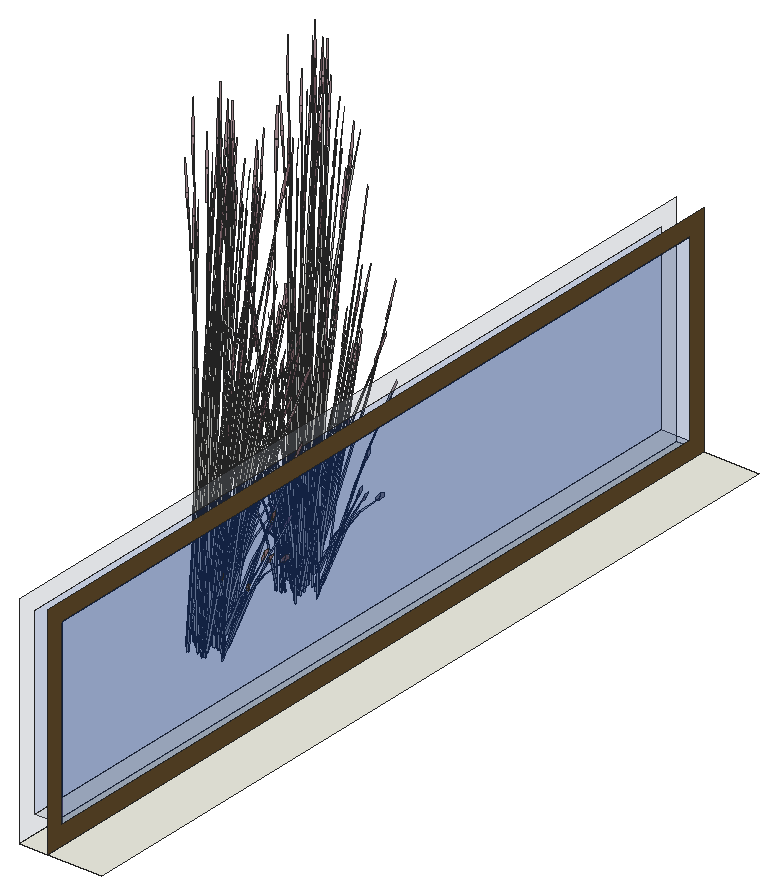
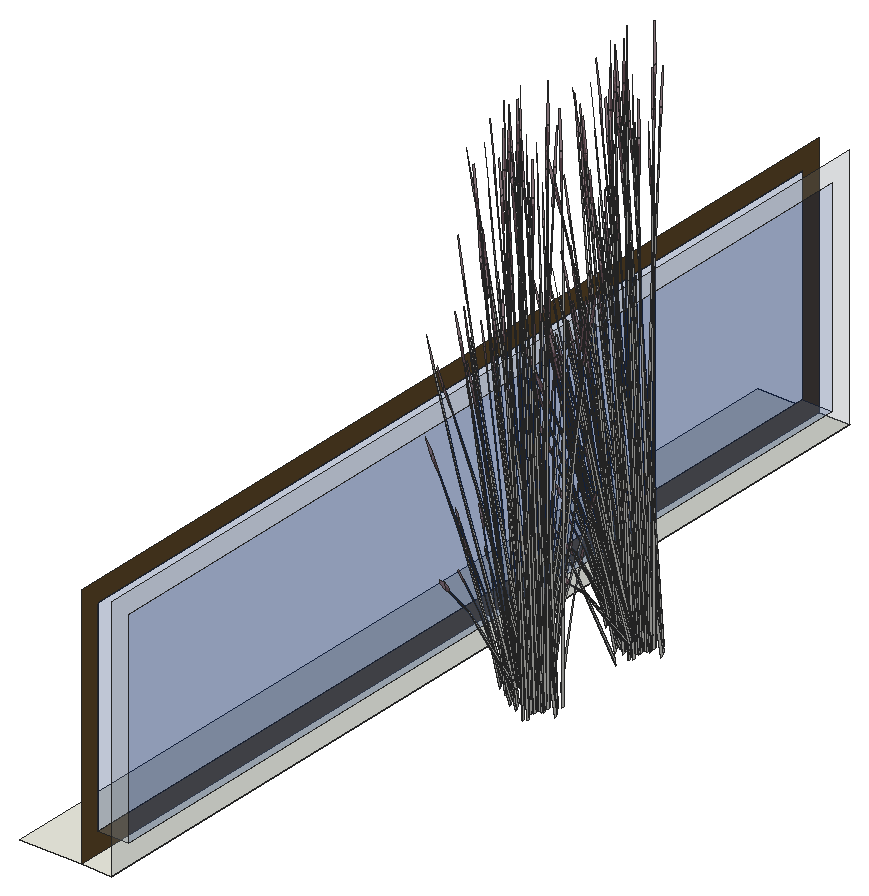
# SketchUp Ruby script. Lengths in inches.
U = 1.inch
M = Sketchup.active_model
def pt(a) = Geom::Point3d.new(a.map { |v| v * U })
def face(e, loops, mat)
  f = e.add_face(loops[0].map { |a| pt(a) })
  loops[1..].each { |l| e.add_face(l.map { |a| pt(a) }).erase! }
  f.material = f.back_material = mat if mat
  f
end
# faces: each face lists its corners as indices into pts; further lists are holes
def faces(e, pts, list, mat = nil) = list.each { |f| face(e, (f[0].is_a?(Array) ? f : [f]).map { |l| l.map { |i| pts[i] } }, mat) }
# xy, xz, yz: faces in a plane at the given z, y or x. An outline is a flat list of corners, or four numbers for a rectangle; further outlines are holes
def ring(l) = l.size == 4 ? [[l[0], l[1]], [l[2], l[1]], [l[2], l[3]], [l[0], l[3]]] : l.each_slice(2).to_a
def flat(e, list, mat, &to3) = list.each { |f| face(e, (f[0].is_a?(Array) ? f : [f]).map { |l| ring(l).map { |u, v| to3.(u, v) } }, mat) }
def xy(e, z, list, mat = nil) = flat(e, list, mat) { |x, y| [x, y, z] }
def xz(e, y, list, mat = nil) = flat(e, list, mat) { |x, z| [x, y, z] }
def yz(e, x, list, mat = nil) = flat(e, list, mat) { |y, z| [x, y, z] }
def lines(e, pts, list) = list.each { |a, b| e.add_line(pt(pts[a]), pt(pts[b])) }
# prism: a flat outline (further loops are holes) pulled along v
def prism(e, loops, v, mat = nil)
  f = face(e, loops, mat); d = Geom::Vector3d.new(v.map { |x| x * U })
  f.pushpull(f.normal.samedirection?(d) ? d.length : -d.length)
end
def box(e, o, s, mat = nil) = prism(e, [[o, [o[0] + s[0], o[1], o[2]], [o[0] + s[0], o[1] + s[1], o[2]], [o[0], o[1] + s[1], o[2]]]], [0, 0, s[2]], mat)
def at(x, y, z, deg = 0) = Geom::Transformation.translation(pt([x, y, z])) * Geom::Transformation.rotation(ORIGIN, Z_AXIS, deg.degrees)
def axes(o, x, y, z) = Geom::Transformation.new([*x, 0, *y, 0, *z, 0, *pt(o).to_a, 1])
def part(name) = M.definitions.add(name)
# library, detail: a bought-in or finely detailed component or shape, given as its bounding box
def library(name, o, s) = part(name).tap { |d| box(d.entities, o, s) }
def detail(e, o, s) = box(e.add_group.entities, o, s)
def put(e, d, t, mat = nil) = e.add_instance(d, t).tap { |i| i.material = mat if mat }
def group(e, t, mat = nil) = e.add_group.tap { |g| g.transformation = t; g.material = mat if mat }.entities
root = M.entities
M.materials.add("D01_Frost_White").color = [238, 238, 227]
M.materials.add("Glass_Basic_01").color = [161, 173, 186]
M.materials["Glass_Basic_01"].alpha = 0.25
M.materials.add("Glass_Sky Reflection_01").color = [0, 46, 142]
M.materials["Glass_Sky Reflection_01"].alpha = 0.25
M.materials.add("LightPink_Translucent").color = [144, 107, 117]
M.materials["LightPink_Translucent"].alpha = 0.75
M.materials.add("Wood_Veneer_15_1K").color = [103, 79, 44]
c1 = part("blade")
p = [[2.15,0.21,22],[0,0.17,0],[0.09,0.45,0],[2.18,0.31,22],[2.29,0.31,22],[0.38,0.45,0],
  [2.48,0.24,33],[2.49,0.24,33],[2.48,0.22,33]]
faces(c1.entities,p,[[0,1,2,3],[4,5,2,3],[6,3,4,7],[8,0,3,6]])
c2 = part("seeds")
p = [[0.3,-0.1,1.38],[-0.01,-0.03,1.59],[-0.01,-0.03,0.03],[0.14,-0.07,-0.07],[0.29,-0.03,3],[0.15,0.01,3.11]]
faces(c2.entities,p,[[0,1,2,3],[1,0,4,5]],"LightPink_Translucent")
c3 = part("blade with seeds")
put(c3.entities,c1,at(0,0,0))
put(c3.entities,c2,axes([2.4,0.25,30.99],[1.5799,-0.05474,1.17369],[-0.12525,1.92788,0.29478],[-0.07173,-0.02425,1.56792]))
xy(root,156,[[427,586,430,676],[430,586,436,676]],"D01_Frost_White")
xy(root,158,[[427,588,430,674]],"Glass_Basic_01")
yz(root,427,[[[586,156,676,180],[588,158,674,178]]],"Glass_Basic_01")
yz(root,427,[[588,158,674,178]],"Glass_Sky Reflection_01")
yz(root,430,[[588,158,674,178]],"Glass_Sky Reflection_01")
yz(root,430,[[[586,156,676,180],[588,158,674,178]]],"Wood_Veneer_15_1K")
put(root,c3,axes([417.75,623.51,155.72],[-0.19883,0.425,-0.37796],[-0.41314,-0.20454,0.1819],[0,0.09797,1.2135]))
put(root,c3,axes([417.54,634.06,158.27],[0.30197,-0.1603,0.05432],[0.1478,0.29231,0.42765],[-0.02916,-0.12885,0.65209]))
put(root,c3,axes([416.5625,625.95,157.83],[0.05195,0.07595,1.47793],[0.41921,0.02984,-0.23373],[0.04216,0.1675,0.11853]))
put(root,c3,axes([418.54,623.25,155.94],[-0.32198,-0.34356,0.14904],[0.32447,-0.33323,0.29641],[-0.03556,0.07016,1.35512]))
put(root,c3,axes([418.54,636.21,156.37],[-0.32198,-0.34356,0.14904],[0.32447,-0.33323,0.29641],[-0.03556,0.07016,1.35512]))
put(root,c3,axes([417.43,623.05,155.71],[0,-0.54574,0],[0.51243,0,0],[0,0,1.51605]))
put(root,c3,axes([417.43,636.01,156.14],[0,-0.54574,0],[0.51243,0,0],[0,0,1.51605]))
put(root,c3,axes([417.43,634.09,158.27],[0.4038,0.12331,0.40553],[-0.13808,0.40538,0.33437],[-0.02427,-0.15942,0.83914]))
put(root,c3,axes([416.95,623.15,155.91],[0.46174,0.2286,0.2033],[-0.22222,0.475,0.42242],[0,-0.1095,1.35626]))
put(root,c3,axes([416.95,636.11,156.33],[0.46174,0.2286,0.2033],[-0.22222,0.475,0.42242],[0,-0.1095,1.35626]))
put(root,c3,axes([417.68,623.27,155.79],[0,0.54548,-0.04762],[-0.51243,0,0],[0,0.01714,1.5153]))
put(root,c3,axes([417.68,636.23,156.21],[0,0.54548,-0.04762],[-0.51243,0,0],[0,0.01714,1.5153]))
put(root,c3,axes([416.8,622.83,156.15],[-0.44501,0.02912,0.37796],[-0.04024,-0.48332,-0.1819],[0.07967,-0.04899,1.2135]))
put(root,c3,axes([416.8,635.79,156.57],[-0.44501,0.02912,0.37796],[-0.04024,-0.48332,-0.1819],[0.07967,-0.04899,1.2135]))
put(root,c3,axes([416.78,624.93,158.12],[0.12355,-0.36271,0.29918],[0.36044,0.10579,-0.38624],[0.03305,0.14603,0.73904]))
put(root,c3,axes([416.59,622,155.94],[-0.11838,0.46875,0.14904],[-0.43321,-0.13265,0.29641],[0.07483,-0.00228,1.35512]))
put(root,c3,axes([416.59,634.96,156.37],[-0.11838,0.46875,0.14904],[-0.43321,-0.13265,0.29641],[0.07483,-0.00228,1.35512]))
put(root,c3,axes([417.44,624.32,155.79],[0.17817,0.54185,-0.05079],[-0.50909,0.18987,0],[0.00622,0.01892,1.45452]))
put(root,c3,axes([417.44,637.28,156.21],[0.17817,0.54185,-0.05079],[-0.50909,0.18987,0],[0.00622,0.01892,1.45452]))
put(root,c3,axes([416.38,634.38,156.28],[-0.25622,-0.47263,0],[0.42866,-0.26357,-0.43598],[0.09763,-0.06003,1.38303]))
put(root,c3,axes([416.85,624.98,158.06],[0.19559,0.38351,-0.60019],[-0.40262,0.21373,0.07243],[0.04574,0.1853,0.84903]))
put(root,c3,axes([418.91,623.61,155.71],[-0.51218,-0.00377,-0.04204],[0,-0.52715,0.42192],[-0.0161,0.12,1.33776]))
put(root,c3,axes([417.91,622.03,155.94],[-0.44036,0.12519,0.14904],[-0.10874,-0.46588,0.29641],[0.03927,0.06788,1.35512]))
put(root,c3,axes([417.91,634.99,156.37],[-0.44036,0.12519,0.14904],[-0.10874,-0.46588,0.29641],[0.03927,0.06788,1.35512]))
put(root,c3,axes([417.46,633.24,156.61],[0.05257,0.27504,0.97034],[-0.29163,-0.15233,0.71294],[0.03138,-0.14083,0.21373]))
put(root,c3,axes([417.26,626.22,158.62],[0.28319,-0.27058,-0.05481],[0.25948,0.29635,-0.2485],[0.01827,0.08397,0.81966]))
put(root,c3,axes([417.18,622.7,155.85],[-0.33979,0.42804,0.38653],[-0.40368,-0.37784,0.15168],[0.08192,-0.04272,1.34202]))
put(root,c3,axes([417.18,635.66,156.27],[-0.33979,0.42804,0.38653],[-0.40368,-0.37784,0.15168],[0.08192,-0.04272,1.34202]))
put(root,c3,axes([417.77,623.38,155.72],[0.28606,0.30466,0],[-0.28606,0.30466,0],[0,0,1.42996]))
put(root,c3,axes([417.77,636.34,156.15],[0.28606,0.30466,0],[-0.28606,0.30466,0],[0,0,1.42996]))
put(root,c3,axes([417.76,623.02,156.15],[0.19883,-0.425,0.37796],[0.41314,0.20454,-0.1819],[0,0.09797,1.2135]))
put(root,c3,axes([417.76,635.98,156.57],[0.19883,-0.425,0.37796],[0.41314,0.20454,-0.1819],[0,0.09797,1.2135]))
put(root,c3,axes([417.59,624.5,155.71],[0.41314,0.21175,0],[-0.19883,0.43999,0],[0,0,1.47801]))
put(root,c3,axes([417.59,637.46,156.14],[0.41314,0.21175,0],[-0.19883,0.43999,0],[0,0,1.47801]))
put(root,c3,axes([417,625.06,157.81],[0.40284,0.11824,-0.43168],[-0.13808,0.40538,-0.33437],[0.03694,0.16321,0.82598]))
put(root,c3,axes([416.66,625.08,158.1],[0.40102,-0.2196,-0.10273],[0.19707,0.38974,-0.57019],[0.05291,0.16424,0.8664]))
put(root,c3,axes([417.63,622.92,155.86],[-0.51796,-0.09937,0.41563],[0.10541,-0.56124,0.1631],[0.07569,0.05419,1.44303]))
put(root,c3,axes([417.63,635.88,156.29],[-0.51796,-0.09937,0.41563],[0.10541,-0.56124,0.1631],[0.07569,0.05419,1.44303]))
put(root,c3,axes([418.7,633.6875,158.25],[-0.04162,0.03603,1.49853],[-0.40776,-0.12155,-0.1416],[-0.01476,-0.15722,0.26519]))
put(root,c3,axes([418.38,634.73,158.53],[-0.45039,-0.02337,-0.10273],[0.01231,-0.44247,-0.57019],[0.03129,-0.17041,0.8664]))
put(root,c3,axes([418.8,623.6875,155.56],[-0.28606,0.29428,-0.2617],[-0.28606,-0.29428,0.2617],[0,0.09479,1.17405]))
put(root,c3,axes([417.78,623.17,155.71],[0.45849,0,0],[0,0.4883,0],[0,0,1.50718]))
put(root,c3,axes([417.78,636.13,156.14],[0.45849,0,0],[0,0.4883,0],[0,0,1.50718]))
put(root,c3,axes([418.21,634.8,158.54],[-0.27728,0.24833,0.29918],[-0.26248,-0.28355,-0.38624],[0.03994,-0.14407,0.73904]))
put(root,c3,axes([417.33,622.63,156.15],[-0.24618,-0.39589,0.37796],[0.37289,-0.27878,-0.1819],[0.07967,0.04899,1.2135]))
put(root,c3,axes([417.33,635.59,156.57],[-0.24618,-0.39589,0.37796],[0.37289,-0.27878,-0.1819],[0.07967,0.04899,1.2135]))
put(root,c3,axes([416.89,622.73,156.1],[-0.04775,-0.53819,-0.2458],[0.49736,-0.03254,-0.42242],[0.08758,-0.07169,1.34921]))
put(root,c3,axes([416.89,635.6875,156.53],[-0.04775,-0.53819,-0.2458],[0.49736,-0.03254,-0.42242],[0.08758,-0.07169,1.34921]))
put(root,c3,axes([417.93,623.12,156.0625],[0.38182,-0.13755,0.12232],[0.13371,0.39278,-0.3493],[0,0.08644,1.07074]))
put(root,c3,axes([417.93,636.08,156.49],[0.38182,-0.13755,0.12232],[0.13371,0.39278,-0.3493],[0,0.08644,1.07074]))
put(root,c3,axes([418.08,634.5625,158.23],[-0.29336,-0.31691,-0.43168],[0.3099,-0.27755,-0.33437],[0.04464,-0.16102,0.82598]))
put(root,c3,axes([417.8,623.15,156.1],[0.46151,0.22505,-0.2458],[-0.22222,0.475,-0.42242],[0.0145,0.11662,1.34921]))
put(root,c3,axes([416.82,621.53,155.56],[0.38233,0.1167,-0.2617],[-0.09626,0.41098,0.2617],[0.07708,-0.04739,1.17405]))
put(root,c3,axes([416.82,634.49,155.99],[0.38233,0.1167,-0.2617],[-0.09626,0.41098,0.2617],[0.07708,-0.04739,1.17405]))
put(root,c3,axes([417.88,634,156.46],[-0.11649,0.09547,1.20808],[-0.34886,-0.1671,-0.25981],[0.06467,-0.20781,0.51652]))
put(root,c3,axes([418.8,623.26,155.95],[0,-0.47166,0.41945],[0.45849,0,0],[0,0.10742,1.33059]))
put(root,c3,axes([418.8,636.22,156.37],[0,-0.47166,0.41945],[0.45849,0,0],[0,0.10742,1.33059]))
put(root,c3,axes([419,623.7,155.56],[0,0.47166,-0.41945],[-0.45849,0,0],[0,0.10742,1.33059]))
put(root,c3,axes([417.78,625.13,157.85],[-0.4076,0.10824,0.40553],[-0.07074,-0.4246,0.33437],[0.09586,0.12514,0.83914]))
put(root,c3,axes([416.73,634.31,155.98],[0.38354,-0.23583,-0.41945],[0.22925,0.42288,0],[0.08735,-0.05371,1.33059]))
put(root,c3,axes([417.7,625.21,157.85],[-0.18625,0.29962,0.05432],[-0.26523,-0.17444,0.42765],[0.08575,0.09606,0.65209]))
put(root,c3,axes([417.23,624.22,157.125],[-0.09368,-0.15143,1.44779],[0.43286,-0.12749,0.11706],[0.09783,0.23774,0.61892]))
put(root,c3,axes([417.5,622.52,156.0625],[0.07906,-0.42093,0.12232],[0.38625,0.07307,-0.3493],[0.07029,0.04322,1.07074]))
put(root,c3,axes([417.5,635.48,156.49],[0.07906,-0.42093,0.12232],[0.38625,0.07307,-0.3493],[0.07029,0.04322,1.07074]))
put(root,c3,axes([418.05,621.79,155.95],[-0.38354,-0.23583,0.41945],[0.22925,-0.42288,0],[0.08735,0.05371,1.33059]))
put(root,c3,axes([418.05,634.75,156.37],[-0.38354,-0.23583,0.41945],[0.22925,-0.42288,0],[0.08735,0.05371,1.33059]))
put(root,c3,axes([418.17,634.71,158.48],[0.01066,-0.43628,-0.60019],[0.44902,0.0293,0.07243],[0.04739,-0.18483,0.84903]))
put(root,c3,axes([417.71,624.25,155.7],[0.43024,-0.16003,-0.16218],[0.15118,0.46099,0.00007],[0.04749,-0.01769,1.46908]))
put(root,c3,axes([417.71,637.21,156.12],[0.43024,-0.16003,-0.16218],[0.15118,0.46099,0.00007],[0.04749,-0.01769,1.46908]))
put(root,c3,axes([417.64,624.87,158.12],[-0.06329,-0.37991,0.29918],[0.36182,-0.10032,-0.38624],[0.09718,0.10887,0.73904]))
put(root,c3,axes([417.72,622.88,155.72],[0.24618,0.39589,-0.37796],[-0.37289,0.27878,0.1819],[0.07967,0.04899,1.2135]))
put(root,c3,axes([417.72,635.84,156.14],[0.24618,0.39589,-0.37796],[-0.37289,0.27878,0.1819],[0.07967,0.04899,1.2135]))
put(root,c3,axes([417.88,622.68,157.63],[-0.35411,-0.24507,1.16821],[0.37391,-0.38156,0.50405],[0.11425,0.22994,1.12919]))
put(root,c3,axes([418.35,634.44,158.1],[0.27728,-0.24833,-0.29918],[0.26248,0.28355,0.38624],[0.03994,-0.14407,0.73904]))
put(root,c3,axes([417.29,625.4,157.83],[0.00121,-0.0571,1.49853],[0.35119,-0.25193,-0.1416],[0.12199,0.08992,0.26519]))
put(root,c3,axes([418.46,634.57,158.27],[0.33677,0.02198,0.05432],[-0.00923,0.33185,0.42765],[0.03524,-0.12712,0.65209]))
put(root,c3,axes([418.42,624.68,156.1875],[-0.23074,-0.13562,0.97034],[0.29794,-0.1378,0.71294],[0.08036,0.11673,0.21373]))
put(root,c3,axes([417.6,624.53,156.04],[0.00723,-0.15635,1.20808],[0.34559,-0.17464,-0.25981],[0.10668,0.18713,0.51652]))
put(root,c3,axes([418.79,634.03,158.26],[-0.00396,-0.09387,1.47793],[-0.33411,-0.2713,-0.23373],[0.05166,-0.16446,0.11853]))
put(root,c3,axes([417.19,622.32,155.59],[0.27603,-0.35451,-0.52676],[0.34289,0.32147,-0.13825],[0.11061,-0.08844,1.16273]))
put(root,c3,axes([417.19,635.28,156.02],[0.27603,-0.35451,-0.52676],[0.34289,0.32147,-0.13825],[0.11061,-0.08844,1.16273]))
put(root,c3,axes([418.35,634.54,158.27],[0.29182,0.32181,0.40553],[-0.3099,0.27755,0.33437],[0.05383,-0.15098,0.83914]))
put(root,c3,axes([418.4,622,155.56],[0.09626,0.41098,-0.2617],[-0.38233,0.1167,0.2617],[0.07708,0.04739,1.17405]))
put(root,c3,axes([418.4,634.96,155.99],[0.09626,0.41098,-0.2617],[-0.38233,0.1167,0.2617],[0.07708,0.04739,1.17405]))
put(root,c3,axes([419.12,623.34,155.86],[0.51243,0,0],[0,0.52715,-0.43598],[0,0.12006,1.38303]))
put(root,c3,axes([417.46,622.66,156.1],[0.41376,-0.31314,-0.2458],[0.27514,0.44246,-0.42242],[0.10209,0.04493,1.34921]))
put(root,c3,axes([417.46,635.62,156.53],[0.41376,-0.31314,-0.2458],[0.27514,0.44246,-0.42242],[0.10209,0.04493,1.34921]))
put(root,c3,axes([418.46,625.29,156.1],[-0.26279,-0.01479,0.88755],[0.17355,-0.31417,0.49003],[0.10382,0.11162,0.6962]))
put(root,c3,axes([418.6875,622.6,158.12],[-0.35672,0.06741,0.29918],[-0.09419,-0.38534,-0.38624],[0.10222,-0.1035,0.73904]))
put(root,c3,axes([418.6875,635.5625,158.54],[-0.35672,0.06741,0.29918],[-0.09419,-0.38534,-0.38624],[0.10222,-0.1035,0.73904]))
put(root,c3,axes([417.66,634.49,157.55],[-0.0763,0.16212,1.44779],[-0.3201,-0.3355,0.11706],[0.1444,-0.2091,0.61892]))
put(root,c3,axes([417.61,625.0625,158.1],[0.2442,-0.40372,-0.10273],[0.35364,0.23259,-0.57019],[0.12293,0.11406,0.8664]))
put(root,c3,axes([416.42,622.38,155.2],[-0.40337,0.18883,1.08919],[-0.12839,-0.54182,0.42321],[0.24769,0.00901,1.23883]))
put(root,c3,axes([416.42,635.34,155.62],[-0.40337,0.18883,1.08919],[-0.12839,-0.54182,0.42321],[0.24769,0.00901,1.23883]))
put(root,c3,axes([418.875,635.6,158.53],[-0.37908,-0.26007,-0.10273],[0.21839,-0.37663,-0.57019],[0.1071,-0.13092,0.8664]))
put(root,c3,axes([417.9,624.86,157.81],[0.40438,-0.11212,-0.43168],[0.07074,0.4246,-0.33437],[0.10862,0.12168,0.82598]))
put(root,c3,axes([418.27,621.54,155.86],[0.25622,-0.47263,0],[0.42866,0.26357,-0.43598],[0.09763,0.06003,1.38303]))
put(root,c3,axes([418.27,634.5,156.28],[0.25622,-0.47263,0],[0.42866,0.26357,-0.43598],[0.09763,0.06003,1.38303]))
put(root,c3,axes([418.7,634.29,155.54],[-0.06134,-0.03716,1.48974],[-0.15755,-0.41512,-0.22758],[0.10629,-0.11265,0.25375]))
put(root,c3,axes([418.36,624.35,158.12],[-0.23317,-0.29531,0.29918],[0.26625,-0.27955,-0.38624],[0.13527,0.04253,0.73904]))
put(root,c3,axes([418.36,637.3125,158.54],[-0.23317,-0.29531,0.29918],[0.26625,-0.27955,-0.38624],[0.13527,0.04253,0.73904]))
put(root,c3,axes([418.5,621.83,155.56],[0.38354,0.23583,-0.41945],[-0.22925,0.42288,0],[0.08735,0.05371,1.33059]))
put(root,c3,axes([418.5,634.78,155.98],[0.38354,0.23583,-0.41945],[-0.22925,0.42288,0],[0.08735,0.05371,1.33059]))
put(root,c3,axes([418.57,624.62,157.85],[-0.02064,0.35866,0.05432],[-0.3116,-0.00983,0.42765],[0.11936,0.03753,0.65209]))
put(root,c3,axes([418.48,625.18,155.11],[0.02986,-0.06809,1.48974],[0.37589,-0.20055,-0.22758],[0.11396,0.1038,0.25375]))
put(root,c3,axes([418.6,624.51,157.85],[-0.30217,0.31079,0.40553],[-0.2606,-0.33005,0.33437],[0.14177,0.05733,0.83914]))
put(root,c3,axes([418.6875,635.29,158.23],[-0.10528,-0.43067,-0.43168],[0.39868,-0.07534,-0.33437],[0.11425,-0.11568,0.82598]))
put(root,c3,axes([419.39,624.55,157.17],[-0.07843,-0.39649,-0.0295],[0.37072,-0.09115,-0.13375],[0.07742,0.02514,0.44114]))
put(root,c3,axes([419.39,637.51,157.6],[-0.07843,-0.39649,-0.0295],[0.37072,-0.09115,-0.13375],[0.07742,0.02514,0.44114]))
put(root,c3,axes([418.75,623.53,158.12],[-0.34057,-0.13158,0.29918],[0.09933,-0.38387,-0.38624],[0.13712,-0.0352,0.73904]))
put(root,c3,axes([418.75,636.49,158.54],[-0.34057,-0.13158,0.29918],[0.09933,-0.38387,-0.38624],[0.13712,-0.0352,0.73904]))
put(root,c3,axes([417.94,622.73,155.59],[0.42629,0.07733,-0.52676],[-0.08996,0.47699,-0.13825],[0.12722,0.0578,1.16273]))
put(root,c3,axes([417.94,635.6875,156.02],[0.42629,0.07733,-0.52676],[-0.08996,0.47699,-0.13825],[0.12722,0.0578,1.16273]))
put(root,c3,axes([419.76,623.01,155.76],[-0.25407,-0.3016,-0.05481],[0.27826,-0.27635,-0.2485],[0.07884,-0.01946,0.81966]))
put(root,c3,axes([419.76,635.97,156.1875],[-0.25407,-0.3016,-0.05481],[0.27826,-0.27635,-0.2485],[0.07884,-0.01946,0.81966]))
put(root,c3,axes([419.18,621.47,156.1875],[-0.1365,0.2401,0.97034],[-0.11733,-0.32258,0.71294],[0.11274,-0.08083,0.21373]))
put(root,c3,axes([419.18,634.43,156.61],[-0.1365,0.2401,0.97034],[-0.11733,-0.32258,0.71294],[0.11274,-0.08083,0.21373]))
put(root,c3,axes([419.01,622.54,157.85],[0.28133,0.19836,0.05432],[-0.16379,0.28248,0.42765],[0.0902,-0.09132,0.65209]))
put(root,c3,axes([419.01,635.5,158.27],[0.28133,0.19836,0.05432],[-0.16379,0.28248,0.42765],[0.0902,-0.09132,0.65209]))
put(root,c3,axes([418.93,622.46,157.85],[0.10163,0.43409,0.40553],[-0.39868,0.07534,0.33437],[0.1175,-0.10209,0.83914]))
put(root,c3,axes([418.93,635.42,158.27],[0.10163,0.43409,0.40553],[-0.39868,0.07534,0.33437],[0.1175,-0.10209,0.83914]))
put(root,c3,axes([417.86,623.75,157.125],[-0.15222,-0.08126,1.44779],[0.31502,-0.34091,0.11706],[0.19634,0.15379,0.61892]))
put(root,c3,axes([419.81,635.49,158.25],[-0.05353,-0.00358,1.49853],[-0.22227,-0.38383,-0.1416],[0.08926,-0.1262,0.26519]))
put(root,c3,axes([418.98,622.375,157.68],[0.35672,-0.06741,-0.29918],[0.09419,0.38534,0.38624],[0.10222,-0.1035,0.73904]))
put(root,c3,axes([418.98,635.34,158.1],[0.35672,-0.06741,-0.29918],[0.09419,0.38534,0.38624],[0.10222,-0.1035,0.73904]))
put(root,c3,axes([418.7,635.46,158.48],[0.21406,-0.37215,-0.60019],[0.37511,0.26448,0.07243],[0.12781,-0.13483,0.84903]))
put(root,c3,axes([419.05,623.64,157.85],[0.15051,0.3216,0.05432],[-0.27447,0.15741,0.42765],[0.12099,-0.03106,0.65209]))
put(root,c3,axes([419.05,636.6,158.27],[0.15051,0.3216,0.05432],[-0.27447,0.15741,0.42765],[0.12099,-0.03106,0.65209]))
put(root,c3,axes([418.69,624.51,157.68],[0.23317,0.29531,-0.29918],[-0.26625,0.27955,0.38624],[0.13527,0.04253,0.73904]))
put(root,c3,axes([418.43,624.54,158.1],[0.02194,-0.47967,-0.10273],[0.41546,0.01311,-0.57019],[0.16001,0.03332,0.8664]))
put(root,c3,axes([418.43,637.5,158.53],[0.02194,-0.47967,-0.10273],[0.41546,0.01311,-0.57019],[0.16001,0.03332,0.8664]))
put(root,c3,axes([418.89,623.65,158.1],[-0.20619,-0.42709,-0.10273],[0.36595,-0.20988,-0.57019],[0.15422,-0.05635,0.8664]))
put(root,c3,axes([418.89,636.61,158.53],[-0.20619,-0.42709,-0.10273],[0.36595,-0.20988,-0.57019],[0.15422,-0.05635,0.8664]))
put(root,c3,axes([419.03,623.53,157.85],[-0.11578,0.43006,0.40553],[-0.38064,-0.14706,0.33437],[0.14969,-0.02584,0.83914]))
put(root,c3,axes([419.03,636.49,158.27],[-0.11578,0.43006,0.40553],[-0.38064,-0.14706,0.33437],[0.14969,-0.02584,0.83914]))
put(root,c3,axes([418.79,624.25,157.83],[0.08791,-0.00798,1.47793],[0.24113,-0.36643,-0.23373],[0.15637,0.04837,0.11853]))
put(root,c3,axes([418.79,637.21,158.26],[0.08791,-0.00798,1.47793],[0.24113,-0.36643,-0.23373],[0.15637,0.04837,0.11853]))
put(root,c3,axes([418.87,623.29,157.81],[0.11102,-0.42903,-0.43168],[0.38064,0.14706,-0.33437],[0.15325,-0.03934,0.82598]))
put(root,c3,axes([418.87,636.25,158.23],[0.11102,-0.42903,-0.43168],[0.38064,0.14706,-0.33437],[0.15325,-0.03934,0.82598]))
put(root,c3,axes([419.83,623.5625,156.1875],[-0.2532,0.07787,0.97034],[0.11918,-0.32181,0.71294],[0.13432,0.02202,0.21373]))
put(root,c3,axes([419.83,636.52,156.61],[-0.2532,0.07787,0.97034],[0.11918,-0.32181,0.71294],[0.13432,0.02202,0.21373]))
put(root,c3,axes([419.01,635.12,156.46],[-0.1464,-0.01397,1.20808],[-0.14998,-0.37477,-0.25981],[0.17985,-0.10602,0.51652]))
put(root,c3,axes([419.1,623.48,157.68],[0.34057,0.13158,-0.29918],[-0.09933,0.38387,0.38624],[0.13712,-0.0352,0.73904]))
put(root,c3,axes([419.1,636.44,158.1],[0.34057,0.13158,-0.29918],[-0.09933,0.38387,0.38624],[0.13712,-0.0352,0.73904]))
put(root,c3,axes([418.45,624.3125,158.06],[0.40965,0.01136,-0.60019],[-0.02751,0.47821,0.07243],[0.17355,0.05047,0.84903]))
put(root,c3,axes([418.45,637.27,158.48],[0.40965,0.01136,-0.60019],[-0.02751,0.47821,0.07243],[0.17355,0.05047,0.84903]))
put(root,c3,axes([419.28,623.41,155.53],[-0.26394,0.0566,1.1961],[-0.04201,-0.45055,0.06846],[0.18486,-0.06819,0.68062]))
put(root,c3,axes([419.28,636.37,155.95],[-0.26394,0.0566,1.1961],[-0.04201,-0.45055,0.06846],[0.18486,-0.06819,0.68062]))
put(root,c3,axes([419.57,623.11,155.11],[-0.02142,-0.07161,1.48974],[0.14855,-0.41887,-0.22758],[0.14984,-0.00603,0.25375]))
put(root,c3,axes([419.57,636.07,155.54],[-0.02142,-0.07161,1.48974],[0.14855,-0.41887,-0.22758],[0.14984,-0.00603,0.25375]))
put(root,c3,axes([419.71,624.92,157.83],[-0.03706,-0.04129,1.49853],[0.08106,-0.44261,-0.1416],[0.14596,-0.02828,0.26519]))
put(root,c3,axes([419.71,637.88,158.25],[-0.03706,-0.04129,1.49853],[0.08106,-0.44261,-0.1416],[0.14596,-0.02828,0.26519]))
put(root,c3,axes([418.18,623.01,157.125],[-0.16998,0.01068,1.44779],[0.11276,-0.46299,0.11706],[0.24224,0.02864,0.61892]))
put(root,c3,axes([418.18,635.97,157.55],[-0.16998,0.01068,1.44779],[0.11276,-0.46299,0.11706],[0.24224,0.02864,0.61892]))
put(root,c3,axes([418.8,623.44,158.06],[0.3601,-0.20831,-0.60019],[0.20068,0.4288,0.07243],[0.17399,-0.04871,0.84903]))
put(root,c3,axes([418.8,636.4,158.48],[0.3601,-0.20831,-0.60019],[0.20068,0.4288,0.07243],[0.17399,-0.04871,0.84903]))
put(root,c3,axes([420.01,622.98,157.83],[0.05687,-0.07184,1.47793],[-0.07279,-0.44069,-0.23373],[0.14268,-0.08356,0.11853]))
put(root,c3,axes([420.01,635.94,158.26],[0.05687,-0.07184,1.47793],[-0.07279,-0.44069,-0.23373],[0.14268,-0.08356,0.11853]))
put(root,c3,axes([419.35,624.08,156.04],[-0.0987,-0.116,1.20808],[0.12841,-0.38374,-0.25981],[0.19968,0.05198,0.51652]))
put(root,c3,axes([419.35,637.04,156.46],[-0.0987,-0.116,1.20808],[0.12841,-0.38374,-0.25981],[0.19968,0.05198,0.51652]))
